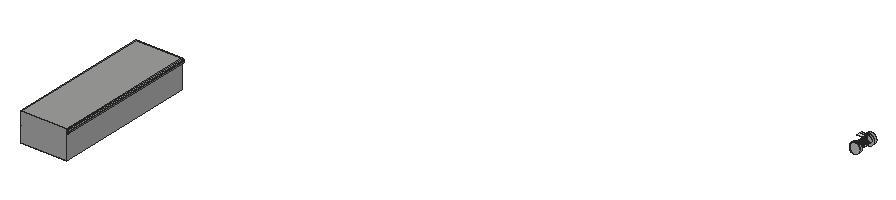
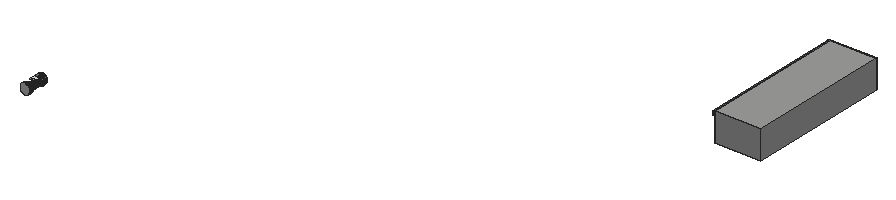
# SketchUp Ruby script. Lengths in inches.
U = 1.inch
M = Sketchup.active_model
def pt(a) = Geom::Point3d.new(a.map { |v| v * U })
def face(e, loops, mat)
  f = e.add_face(loops[0].map { |a| pt(a) })
  loops[1..].each { |l| e.add_face(l.map { |a| pt(a) }).erase! }
  f.material = f.back_material = mat if mat
  f
end
# faces: each face lists its corners as indices into pts; further lists are holes
def faces(e, pts, list, mat = nil) = list.each { |f| face(e, (f[0].is_a?(Array) ? f : [f]).map { |l| l.map { |i| pts[i] } }, mat) }
# xy, xz, yz: faces in a plane at the given z, y or x. An outline is a flat list of corners, or four numbers for a rectangle; further outlines are holes
def ring(l) = l.size == 4 ? [[l[0], l[1]], [l[2], l[1]], [l[2], l[3]], [l[0], l[3]]] : l.each_slice(2).to_a
def flat(e, list, mat, &to3) = list.each { |f| face(e, (f[0].is_a?(Array) ? f : [f]).map { |l| ring(l).map { |u, v| to3.(u, v) } }, mat) }
def xy(e, z, list, mat = nil) = flat(e, list, mat) { |x, y| [x, y, z] }
def xz(e, y, list, mat = nil) = flat(e, list, mat) { |x, z| [x, y, z] }
def yz(e, x, list, mat = nil) = flat(e, list, mat) { |y, z| [x, y, z] }
def lines(e, pts, list) = list.each { |a, b| e.add_line(pt(pts[a]), pt(pts[b])) }
# prism: a flat outline (further loops are holes) pulled along v
def prism(e, loops, v, mat = nil)
  f = face(e, loops, mat); d = Geom::Vector3d.new(v.map { |x| x * U })
  f.pushpull(f.normal.samedirection?(d) ? d.length : -d.length)
end
def box(e, o, s, mat = nil) = prism(e, [[o, [o[0] + s[0], o[1], o[2]], [o[0] + s[0], o[1] + s[1], o[2]], [o[0], o[1] + s[1], o[2]]]], [0, 0, s[2]], mat)
def at(x, y, z, deg = 0) = Geom::Transformation.translation(pt([x, y, z])) * Geom::Transformation.rotation(ORIGIN, Z_AXIS, deg.degrees)
def axes(o, x, y, z) = Geom::Transformation.new([*x, 0, *y, 0, *z, 0, *pt(o).to_a, 1])
def part(name) = M.definitions.add(name)
# library, detail: a bought-in or finely detailed component or shape, given as its bounding box
def library(name, o, s) = part(name).tap { |d| box(d.entities, o, s) }
def detail(e, o, s) = box(e.add_group.entities, o, s)
def put(e, d, t, mat = nil) = e.add_instance(d, t).tap { |i| i.material = mat if mat }
def group(e, t, mat = nil) = e.add_group.tap { |g| g.transformation = t; g.material = mat if mat }.entities
root = M.entities
M.materials.add("[Aluminum]").color = [178, 178, 178]
M.materials.add("crushed-stone-asphalt-staggered-isosceles-2423-mm-architextu").color = [158, 158, 157]
c1 = part("Stair tread")
xy(c1.entities,0,[[0,0,11.5,36]])
xy(c1.entities,7,[[0,0,11.5,36]])
xz(c1.entities,0,[[0,0,11.5,7],[11.5,6,11.63,6.02,11.75,6.07,11.85,6.15,11.93,6.25,11.98,6.37,12,6.5,11.98,6.63,11.93,6.75,11.85,6.85,11.75,6.93,11.63,6.98,11.5,7]])
xz(c1.entities,36,[[0,0,11.5,7],[11.5,6,11.5,7,11.63,6.98,11.75,6.93,11.85,6.85,11.93,6.75,11.98,6.63,12,6.5,11.98,6.37,11.93,6.25,11.85,6.15,11.75,6.07,11.63,6.02]])
yz(c1.entities,0,[[0,0,36,7]])
yz(c1.entities,11.5,[[0,0,36,6],[0,6,10.3125,7],[10.3125,6,36,7]])
p = [[11.5,36,6],[11.63,36,6.02],[11.63,0,6.02],[11.5,0,6],[11.5,10.3125,6],[11.75,36,6.07],
  [11.75,0,6.07],[11.85,36,6.15],[11.85,0,6.15],[11.93,36,6.25],[11.93,0,6.25],[11.98,36,6.37],
  [11.98,0,6.37],[12,36,6.5],[12,0,6.5],[11.98,36,6.63],[11.98,0,6.63],[11.93,36,6.75],
  [11.93,0,6.75],[11.85,36,6.85],[11.85,0,6.85],[11.75,36,6.93],[11.63,36,6.98],[11.63,0,6.98],
  [11.75,0,6.93],[11.5,36,7],[11.5,10.3125,7],[11.5,0,7]]
faces(c1.entities,p,[[0,1,2,3,4],[1,5,6,2],[5,7,8,6],[7,9,10,8],[9,11,12,10],[11,13,14,12],[13,15,16,14],[15,17,18,16],
  [17,19,20,18],[21,22,23,24],[19,21,24,20],[25,26,27,23,22]])
xy(root,65.29,[[211.63,132.28,211.71,133.02]],"[Aluminum]")
xy(root,65.33,[[211.63,127.79,211.71,128.53]],"[Aluminum]")
xy(root,65.58,[[211.65,129.28,211.71,131.53]])
xy(root,65.58,[[211.65,128.53,211.71,129.28],[211.65,131.53,211.71,132.28]],"[Aluminum]")
xy(root,67.55,[[211.65,129.28,211.71,131.53]])
xy(root,67.55,[[211.65,128.53,211.71,129.28],[211.65,131.53,211.71,132.28]],"[Aluminum]")
xy(root,67.8,[[211.63,127.79,211.71,128.53]],"[Aluminum]")
xy(root,67.84,[[211.63,132.28,211.71,133.02]],"[Aluminum]")
xy(root,68.11,[[210.46,130.03,211.84,131.15]])
xy(root,68.11,[[210.46,131.15,211.84,131.53]],"[Aluminum]")
xz(root,127.79,[[211.63,65.33,211.79,65.33,211.95,65.35,212.03,65.37,212.1,65.39,212.17,65.42,212.25,65.46,212.32,65.5,212.38,65.54,212.45,65.58,212.51,65.64,212.57,65.69,212.62,65.75,212.67,65.8125,212.72,65.88,212.76,65.95,212.79,66.02,212.83,66.09,212.85,66.17,212.875,66.25,212.89,66.32,212.91,66.4,212.92,66.48,212.92,66.65,212.91,66.73,212.89,66.81,212.875,66.88,212.85,66.96,212.83,67.04,212.79,67.11,212.76,67.18,212.71,67.25,212.67,67.32,212.62,67.38,212.51,67.49,212.45,67.54,212.38,67.59,212.3125,67.63,212.24,67.67,212.17,67.71,212.1,67.73,212.02,67.76,211.95,67.78,211.79,67.8,211.63,67.8,211.55,67.79,211.48,67.78,211.4,67.76,211.32,67.73,211.18,67.67,211.04,67.59,210.92,67.49,210.86,67.4375,210.81,67.38,210.76,67.32,210.71,67.25,210.63,67.11,210.6,67.04,210.57,66.96,210.53,66.8,210.51,66.64,210.51,66.48,210.53,66.32,210.55,66.24,210.57,66.17,210.6,66.09,210.63,66.02,210.71,65.88,210.76,65.8125,210.81,65.75,210.86,65.69,210.92,65.63,210.98,65.58,211.04,65.54,211.11,65.49,211.18,65.46,211.25,65.42,211.33,65.39,211.4,65.37,211.48,65.35,211.56,65.34]],"[Aluminum]")
xz(root,128.53,[[[211.63,65.33,211.56,65.34,211.48,65.35,211.4,65.37,211.33,65.39,211.25,65.42,211.18,65.46,211.11,65.49,211.04,65.54,210.98,65.58,210.92,65.63,210.86,65.69,210.81,65.75,210.76,65.8125,210.71,65.88,210.63,66.02,210.6,66.09,210.57,66.17,210.55,66.24,210.53,66.32,210.51,66.48,210.51,66.64,210.53,66.8,210.57,66.96,210.6,67.04,210.63,67.11,210.71,67.25,210.76,67.32,210.81,67.38,210.86,67.4375,210.92,67.49,211.04,67.59,211.18,67.67,211.32,67.73,211.4,67.76,211.48,67.78,211.55,67.79,211.63,67.8,211.79,67.8,211.95,67.78,212.02,67.76,212.1,67.73,212.17,67.71,212.24,67.67,212.3125,67.63,212.38,67.59,212.45,67.54,212.51,67.49,212.62,67.38,212.67,67.32,212.71,67.25,212.76,67.18,212.79,67.11,212.83,67.04,212.85,66.96,212.875,66.88,212.89,66.81,212.91,66.73,212.92,66.65,212.92,66.48,212.91,66.4,212.89,66.32,212.875,66.25,212.85,66.17,212.83,66.09,212.79,66.02,212.76,65.95,212.72,65.88,212.67,65.8125,212.62,65.75,212.57,65.69,212.51,65.64,212.45,65.58,212.38,65.54,212.32,65.5,212.25,65.46,212.17,65.42,212.1,65.39,212.03,65.37,211.95,65.35,211.79,65.33],[211.65,65.58,211.78,65.58,211.96,65.61,212.02,65.63,212.08,65.66,212.14,65.68,212.19,65.71,212.25,65.75,212.3,65.78,212.35,65.82,212.39,65.87,212.44,65.92,212.48,65.97,212.51,66.02,212.55,66.07,212.57,66.13,212.6,66.1875,212.625,66.25,212.64,66.31,212.66,66.37,212.67,66.4375,212.67,66.69,212.66,66.76,212.64,66.82,212.625,66.88,212.6,66.94,212.57,67,212.55,67.06,212.51,67.11,212.48,67.16,212.44,67.21,212.35,67.3,212.25,67.38,212.19,67.42,212.14,67.45,212.08,67.47,212.02,67.5,211.96,67.51,211.9,67.53,211.78,67.55,211.65,67.55,211.53,67.53,211.46,67.51,211.4,67.5,211.34,67.47,211.29,67.45,211.23,67.42,211.03,67.26,210.91,67.11,210.88,67.06,210.82,66.94,210.78,66.82,210.77,66.76,210.76,66.69,210.75,66.63,210.75,66.5,210.76,66.4375,210.77,66.37,210.78,66.31,210.8,66.25,210.82,66.1875,210.85,66.13,210.88,66.07,210.91,66.02,211.03,65.87,211.08,65.82,211.13,65.78,211.18,65.75,211.23,65.71,211.29,65.68,211.34,65.66,211.4,65.63,211.46,65.61,211.53,65.6]]],"[Aluminum]")
xz(root,132.28,[[[211.63,65.29,211.79,65.29,211.96,65.31,212.04,65.33,212.11,65.35,212.19,65.38,212.26,65.42,212.34,65.46,212.41,65.5,212.47,65.55,212.54,65.6,212.6,65.66,212.65,65.72,212.7,65.79,212.75,65.85,212.79,65.93,212.83,66,212.87,66.08,212.89,66.15,212.92,66.23,212.9375,66.31,212.95,66.4,212.96,66.48,212.96,66.65,212.95,66.73,212.9375,66.8125,212.92,66.9,212.89,66.98,212.87,67.05,212.83,67.13,212.75,67.27,212.65,67.41,212.59,67.47,212.54,67.53,212.47,67.58,212.41,67.63,212.34,67.67,212.26,67.71,212.19,67.75,212.11,67.78,212.04,67.8,211.96,67.82,211.79,67.84,211.63,67.84,211.47,67.82,211.39,67.8,211.3125,67.78,211.23,67.75,211.02,67.63,210.95,67.58,210.89,67.53,210.77,67.41,210.67,67.27,210.59,67.13,210.56,67.05,210.53,66.98,210.51,66.89,210.49,66.8125,210.48,66.73,210.47,66.65,210.46,66.5625,210.47,66.48,210.48,66.4,210.49,66.3125,210.51,66.23,210.53,66.15,210.56,66.07,210.59,66,210.63,65.92,210.68,65.85,210.72,65.79,210.77,65.72,210.89,65.6,210.95,65.55,211.02,65.5,211.16,65.42,211.24,65.38,211.3125,65.35,211.39,65.33,211.47,65.31],[211.65,65.58,211.53,65.6,211.46,65.61,211.4,65.63,211.34,65.66,211.29,65.68,211.23,65.71,211.18,65.75,211.13,65.78,211.08,65.82,211.03,65.87,210.91,66.02,210.88,66.07,210.85,66.13,210.82,66.1875,210.8,66.25,210.78,66.31,210.77,66.37,210.76,66.4375,210.75,66.5,210.75,66.63,210.76,66.69,210.77,66.76,210.78,66.82,210.82,66.94,210.88,67.06,210.91,67.11,211.03,67.26,211.23,67.42,211.29,67.45,211.34,67.47,211.4,67.5,211.46,67.51,211.53,67.53,211.65,67.55,211.78,67.55,211.9,67.53,211.96,67.51,212.02,67.5,212.08,67.47,212.14,67.45,212.19,67.42,212.25,67.38,212.35,67.3,212.44,67.21,212.48,67.16,212.51,67.11,212.55,67.06,212.57,67,212.6,66.94,212.625,66.88,212.64,66.82,212.66,66.76,212.67,66.69,212.67,66.4375,212.66,66.37,212.64,66.31,212.625,66.25,212.6,66.1875,212.57,66.13,212.55,66.07,212.51,66.02,212.48,65.97,212.44,65.92,212.39,65.87,212.35,65.82,212.3,65.78,212.25,65.75,212.19,65.71,212.14,65.68,212.08,65.66,212.02,65.63,211.96,65.61,211.78,65.58]]],"[Aluminum]")
xz(root,133.02,[[211.63,65.29,211.47,65.31,211.39,65.33,211.3125,65.35,211.24,65.38,211.16,65.42,211.02,65.5,210.95,65.55,210.89,65.6,210.77,65.72,210.72,65.79,210.68,65.85,210.63,65.92,210.59,66,210.56,66.07,210.53,66.15,210.51,66.23,210.49,66.3125,210.48,66.4,210.47,66.48,210.46,66.5625,210.47,66.65,210.48,66.73,210.49,66.8125,210.51,66.89,210.53,66.98,210.56,67.05,210.59,67.13,210.67,67.27,210.77,67.41,210.89,67.53,210.95,67.58,211.02,67.63,211.23,67.75,211.3125,67.78,211.39,67.8,211.47,67.82,211.63,67.84,211.79,67.84,211.96,67.82,212.04,67.8,212.11,67.78,212.19,67.75,212.26,67.71,212.34,67.67,212.41,67.63,212.47,67.58,212.54,67.53,212.59,67.47,212.65,67.41,212.75,67.27,212.83,67.13,212.87,67.05,212.89,66.98,212.92,66.9,212.9375,66.8125,212.95,66.73,212.96,66.65,212.96,66.48,212.95,66.4,212.9375,66.31,212.92,66.23,212.89,66.15,212.87,66.08,212.83,66,212.79,65.93,212.75,65.85,212.7,65.79,212.65,65.72,212.6,65.66,212.54,65.6,212.47,65.55,212.41,65.5,212.34,65.46,212.26,65.42,212.19,65.38,212.11,65.35,212.04,65.33,211.96,65.31,211.79,65.29]],"[Aluminum]")
yz(root,210.51,[[127.79,66.48,128.53,66.5625],[127.79,66.5625,128.53,66.64]],"[Aluminum]")
yz(root,210.75,[[129.28,66.5,131.53,66.5625],[129.28,66.5625,131.53,66.63]])
yz(root,210.75,[[128.53,66.5,129.28,66.5625],[131.53,66.5,132.28,66.5625],[128.53,66.5625,129.28,66.63],[131.53,66.5625,132.28,66.63]],"[Aluminum]")
p = [[211.48,128.53,65.35],[211.56,128.53,65.34],[211.56,127.79,65.34],[211.48,127.79,65.35],[211.63,128.53,65.33],[211.63,127.79,65.33],
  [211.39,132.28,65.33],[211.3125,132.28,65.35],[211.3125,133.02,65.35],[211.39,133.02,65.33],[211.47,132.28,65.31],[211.47,133.02,65.31],
  [211.55,132.28,65.3],[211.55,133.02,65.3],[211.63,132.28,65.29],[211.63,133.02,65.29],[211.18,128.53,65.46],[211.25,128.53,65.42],
  [211.25,127.79,65.42],[211.18,127.79,65.46],[211.33,128.53,65.39],[211.33,127.79,65.39],[211.4,128.53,65.37],[211.4,127.79,65.37],
  [211.16,132.28,65.42],[211.09,132.28,65.46],[211.09,133.02,65.46],[211.16,133.02,65.42],[211.24,132.28,65.38],[211.24,133.02,65.38],
  [210.98,128.53,65.58],[211.04,128.53,65.54],[211.04,127.79,65.54],[210.98,127.79,65.58],[211.11,128.53,65.49],[211.11,127.79,65.49],
  [210.95,132.28,65.55],[210.89,132.28,65.6],[210.89,133.02,65.6],[210.95,133.02,65.55],[211.02,132.28,65.5],[211.02,133.02,65.5],
  [210.86,128.53,65.69],[210.92,128.53,65.63],[210.92,127.79,65.63],[210.86,127.79,65.69],[211.4,129.28,65.63],[211.34,129.28,65.66],
  [211.34,128.53,65.66],[211.4,128.53,65.63],[211.46,129.28,65.61],[211.46,128.53,65.61],[211.53,129.28,65.6],[211.53,128.53,65.6],
  [211.59,129.28,65.59],[211.59,128.53,65.59],[211.65,129.28,65.58],[211.65,128.53,65.58],[211.34,131.53,65.66],[211.4,131.53,65.63],
  [211.46,131.53,65.61],[211.53,131.53,65.6],[211.59,131.53,65.59],[211.65,131.53,65.58],[211.34,132.28,65.66],[211.4,132.28,65.63],
  [211.46,132.28,65.61],[211.53,132.28,65.6],[211.59,132.28,65.59],[211.65,132.28,65.58],[210.83,132.28,65.66],[210.83,133.02,65.66],
  [210.76,128.53,65.8125],[210.81,128.53,65.75],[210.81,127.79,65.75],[210.76,127.79,65.8125],[211.18,129.28,65.75],[211.13,129.28,65.78],
  [211.13,128.53,65.78],[211.18,128.53,65.75],[211.23,129.28,65.71],[211.23,128.53,65.71],[211.29,129.28,65.68],[211.29,128.53,65.68],
  [211.13,131.53,65.78],[211.18,131.53,65.75],[211.23,131.53,65.71],[211.29,131.53,65.68],[211.13,132.28,65.78],[211.18,132.28,65.75],
  [211.23,132.28,65.71],[211.29,132.28,65.68],[210.77,132.28,65.72],[210.72,132.28,65.79],[210.72,133.02,65.79],[210.77,133.02,65.72],
  [210.71,128.53,65.88],[210.71,127.79,65.88],[211.08,129.28,65.82],[211.03,129.28,65.87],[211.03,128.53,65.87],[211.08,128.53,65.82],
  [211.03,131.53,65.87],[211.08,131.53,65.82],[211.03,132.28,65.87],[211.08,132.28,65.82],[210.68,132.28,65.85],[210.68,133.02,65.85],
  [210.63,128.53,66.02],[210.67,128.53,65.95],[210.67,127.79,65.95],[210.63,127.79,66.02],[210.99,129.28,65.92],[210.95,129.28,65.97],
  [210.95,128.53,65.97],[210.99,128.53,65.92],[210.95,131.53,65.97],[210.99,131.53,65.92],[210.95,132.28,65.97],[210.99,132.28,65.92],
  [210.63,132.28,65.92],[210.59,132.28,66],[210.59,133.02,66],[210.63,133.02,65.92],[210.6,128.53,66.09],[210.6,127.79,66.09],
  [210.91,129.28,66.02],[210.88,129.28,66.07],[210.88,128.53,66.07],[210.91,128.53,66.02],[210.88,131.53,66.07],[210.91,131.53,66.02],
  [210.88,132.28,66.07],[210.91,132.28,66.02],[210.56,132.28,66.07],[210.56,133.02,66.07],[210.57,128.53,66.17],[210.57,127.79,66.17],
  [210.85,129.28,66.13],[210.82,129.28,66.1875],[210.82,128.53,66.1875],[210.85,128.53,66.13],[210.82,131.53,66.1875],[210.85,131.53,66.13],
  [210.82,132.28,66.1875],[210.85,132.28,66.13],[210.53,132.28,66.15],[210.53,133.02,66.15],[210.53,128.53,66.32],[210.55,128.53,66.24],
  [210.55,127.79,66.24],[210.53,127.79,66.32],[210.8,129.28,66.25],[210.78,129.28,66.31],[210.78,128.53,66.31],[210.8,128.53,66.25],
  [210.78,131.53,66.31],[210.8,131.53,66.25],[210.78,132.28,66.31],[210.8,132.28,66.25],[210.51,132.28,66.23],[210.49,132.28,66.3125],
  [210.49,133.02,66.3125],[210.51,133.02,66.23],[210.52,128.53,66.4],[210.52,127.79,66.4],[210.77,129.28,66.37],[210.77,128.53,66.37],
  [210.77,131.53,66.37],[210.77,132.28,66.37],[210.48,132.28,66.4],[210.48,133.02,66.4],[210.51,128.53,66.48],[210.51,127.79,66.48],
  [210.76,129.28,66.4375],[210.75,129.28,66.5],[210.75,128.53,66.5],[210.76,128.53,66.4375],[210.75,131.53,66.5],[210.76,131.53,66.4375],
  [210.75,132.28,66.5],[210.76,132.28,66.4375],[210.47,132.28,66.48],[210.47,133.02,66.48],[210.46,132.28,66.5625],[210.46,133.02,66.5625],
  [210.52,128.53,66.72],[210.51,128.53,66.64],[210.51,127.79,66.64],[210.52,127.79,66.72],[210.75,129.28,66.63],[210.76,129.28,66.69],
  [210.76,128.53,66.69],[210.75,128.53,66.63],[210.76,131.53,66.69],[210.75,131.53,66.63],[210.76,132.28,66.69],[210.75,132.28,66.63],
  [210.47,132.28,66.65],[210.47,133.02,66.65],[210.48,132.28,66.73],[210.48,133.02,66.73],[210.53,128.53,66.8],[210.53,127.79,66.8],
  [210.77,129.28,66.76],[210.77,128.53,66.76],[210.77,131.53,66.76],[210.77,132.28,66.76],[210.49,132.28,66.8125],[210.49,133.02,66.8125],
  [210.55,128.53,66.88],[210.55,127.79,66.88],[210.78,129.28,66.82],[210.78,128.53,66.82],[210.8,129.28,66.88],[210.8,128.53,66.88],
  [210.78,131.53,66.82],[210.8,131.53,66.88],[210.78,132.28,66.82],[210.8,132.28,66.88],[210.51,132.28,66.89],[210.51,133.02,66.89],
  [210.57,128.53,66.96],[210.57,127.79,66.96],[210.82,129.28,66.94],[210.82,128.53,66.94],[210.85,129.28,67],[210.85,128.53,67],
  [210.82,131.53,66.94],[210.85,131.53,67],[210.82,132.28,66.94],[210.85,132.28,67],[210.53,132.28,66.98],[210.53,133.02,66.98],
  [210.6,128.53,67.04],[210.6,127.79,67.04],[210.63,128.53,67.11],[210.63,127.79,67.11],[210.88,129.28,67.06],[210.88,128.53,67.06],
  [210.88,131.53,67.06],[210.88,132.28,67.06],[210.56,132.28,67.05],[210.56,133.02,67.05],[210.67,128.53,67.18],[210.67,127.79,67.18],
  [210.91,129.28,67.11],[210.91,128.53,67.11],[210.95,129.28,67.16],[210.95,128.53,67.16],[210.91,131.53,67.11],[210.95,131.53,67.16],
  [210.91,132.28,67.11],[210.95,132.28,67.16],[210.59,132.28,67.13],[210.59,133.02,67.13],[210.63,132.28,67.2],[210.63,133.02,67.2],
  [210.71,128.53,67.25],[210.71,127.79,67.25],[210.76,128.53,67.32],[210.76,127.79,67.32],[210.99,129.28,67.21],[210.99,128.53,67.21],
  [211.03,129.28,67.26],[211.03,128.53,67.26],[210.99,131.53,67.21],[211.03,131.53,67.26],[210.99,132.28,67.21],[211.03,132.28,67.26],
  [210.67,132.28,67.27],[210.67,133.02,67.27],[210.81,128.53,67.38],[210.81,127.79,67.38],[211.08,129.28,67.3],[211.08,128.53,67.3],
  [211.13,129.28,67.34],[211.13,128.53,67.34],[211.18,129.28,67.38],[211.18,128.53,67.38],[211.08,131.53,67.3],[211.13,131.53,67.34],
  [211.18,131.53,67.38],[211.08,132.28,67.3],[211.13,132.28,67.34],[211.18,132.28,67.38],[210.72,132.28,67.34],[210.72,133.02,67.34],
  [210.77,132.28,67.41],[210.77,133.02,67.41],[210.86,128.53,67.4375],[210.86,127.79,67.4375],[210.92,128.53,67.49],[210.92,127.79,67.49],
  [211.23,129.28,67.42],[211.23,128.53,67.42],[211.29,129.28,67.45],[211.29,128.53,67.45],[211.34,129.28,67.47],[211.34,128.53,67.47],
  [211.23,131.53,67.42],[211.29,131.53,67.45],[211.34,131.53,67.47],[211.23,132.28,67.42],[211.29,132.28,67.45],[211.34,132.28,67.47],
  [210.83,132.28,67.47],[210.83,133.02,67.47],[210.98,128.53,67.54],[210.98,127.79,67.54],[211.04,128.53,67.59],[211.04,127.79,67.59],
  [211.4,129.28,67.5],[211.4,128.53,67.5],[211.46,129.28,67.51],[211.46,128.53,67.51],[211.53,129.28,67.53],[211.53,128.53,67.53],
  [211.59,129.28,67.54],[211.59,128.53,67.54],[211.65,129.28,67.55],[211.65,128.53,67.55],[211.4,131.53,67.5],[211.46,131.53,67.51],
  [211.53,131.53,67.53],[211.59,131.53,67.54],[211.65,131.53,67.55],[211.4,132.28,67.5],[211.46,132.28,67.51],[211.53,132.28,67.53],
  [211.59,132.28,67.54],[211.65,132.28,67.55],[210.89,132.28,67.53],[210.89,133.02,67.53],[210.95,132.28,67.58],[210.95,133.02,67.58],
  [211.11,128.53,67.63],[211.11,127.79,67.63],[211.18,128.53,67.67],[211.18,127.79,67.67],[211.02,132.28,67.63],[211.02,133.02,67.63],
  [211.09,132.28,67.67],[211.09,133.02,67.67],[211.25,128.53,67.7],[211.25,127.79,67.7],[211.32,128.53,67.73],[211.32,127.79,67.73],
  [211.4,128.53,67.76],[211.4,127.79,67.76],[211.16,132.28,67.71],[211.16,133.02,67.71],[211.23,132.28,67.75],[211.23,133.02,67.75],
  [211.3125,132.28,67.78],[211.3125,133.02,67.78],[211.48,128.53,67.78],[211.48,127.79,67.78],[211.55,128.53,67.79],[211.55,127.79,67.79],
  [211.63,128.53,67.8],[211.63,127.79,67.8],[211.39,132.28,67.8],[211.39,133.02,67.8],[211.47,132.28,67.82],[211.47,133.02,67.82],
  [211.55,132.28,67.83],[211.55,133.02,67.83],[211.63,132.28,67.84],[211.63,133.02,67.84]]
faces(root,p,[[0,1,2,3],[1,4,5,2],[6,7,8,9],[10,6,9,11],[12,10,11,13],[14,12,13,15],[16,17,18,19],[17,20,21,18],
  [20,22,23,21],[22,0,3,23],[24,25,26,27],[28,24,27,29],[7,28,29,8],[30,31,32,33],[31,34,35,32],[34,16,19,35],
  [36,37,38,39],[40,36,39,41],[25,40,41,26],[42,43,44,45],[43,30,33,44],[46,47,48,49],[50,46,49,51],[52,50,51,53],
  [54,52,53,55],[56,54,55,57],[59,58,64,65],[60,59,65,66],[61,60,66,67],[62,61,67,68],[63,62,68,69],[37,70,71,38],
  [72,73,74,75],[73,42,45,74],[76,77,78,79],[80,76,79,81],[82,80,81,83],[47,82,83,48],[85,84,88,89],[86,85,89,90],
  [87,86,90,91],[58,87,91,64],[92,93,94,95],[70,92,95,71],[96,72,75,97],[98,99,100,101],[77,98,101,78],[103,102,104,105],
  [84,103,105,88],[93,106,107,94],[108,109,110,111],[109,96,97,110],[112,113,114,115],[99,112,115,100],[117,116,118,119],[102,117,119,104],
  [120,121,122,123],[106,120,123,107],[124,108,111,125],[126,127,128,129],[113,126,129,114],[131,130,132,133],[116,131,133,118],[121,134,135,122],
  [136,124,125,137],[138,139,140,141],[127,138,141,128],[143,142,144,145],[130,143,145,132],[134,146,147,135],[148,149,150,151],[149,136,137,150],
  [152,153,154,155],[139,152,155,140],[157,156,158,159],[142,157,159,144],[160,161,162,163],[146,160,163,147],[164,148,151,165],[153,166,167,154],
  [156,168,169,158],[161,170,171,162],[172,164,165,173],[174,175,176,177],[166,174,177,167],[179,178,180,181],[168,179,181,169],[170,182,183,171],
  [182,184,185,183],[186,187,188,189],[190,191,192,193],[195,194,196,197],[184,198,199,185],[198,200,201,199],[202,186,189,203],[191,204,205,192],
  [194,206,207,196],[200,208,209,201],[210,202,203,211],[204,212,213,205],[212,214,215,213],[206,216,218,207],[216,217,219,218],[208,220,221,209],
  [222,210,211,223],[214,224,225,215],[224,226,227,225],[217,228,230,219],[228,229,231,230],[220,232,233,221],[234,222,223,235],[236,234,235,237],
  [226,238,239,227],[229,240,241,231],[232,242,243,233],[244,236,237,245],[238,246,247,239],[246,248,249,247],[240,250,252,241],[250,251,253,252],
  [242,254,255,243],[254,256,257,255],[258,244,245,259],[260,258,259,261],[248,262,263,249],[262,264,265,263],[251,266,268,253],[266,267,269,268],
  [256,270,271,257],[272,260,261,273],[264,274,275,265],[274,276,277,275],[276,278,279,277],[267,280,283,269],[280,281,284,283],[281,282,285,284],
  [270,286,287,271],[286,288,289,287],[290,272,273,291],[292,290,291,293],[278,294,295,279],[294,296,297,295],[296,298,299,297],[282,300,303,285],
  [300,301,304,303],[301,302,305,304],[288,306,307,289],[308,292,293,309],[310,308,309,311],[298,312,313,299],[312,314,315,313],[314,316,317,315],
  [316,318,319,317],[318,320,321,319],[302,322,327,305],[322,323,328,327],[323,324,329,328],[324,325,330,329],[325,326,331,330],[306,332,333,307],
  [332,334,335,333],[336,310,311,337],[338,336,337,339],[334,340,341,335],[340,342,343,341],[344,338,339,345],[346,344,345,347],[348,346,347,349],
  [342,350,351,343],[350,352,353,351],[352,354,355,353],[356,348,349,357],[358,356,357,359],[360,358,359,361],[354,362,363,355],[362,364,365,363],
  [364,366,367,365],[366,368,369,367]],"[Aluminum]")
faces(root,p,[[58,59,46,47],[59,60,50,46],[60,61,52,50],[61,62,54,52],[62,63,56,54],[84,85,76,77],[85,86,80,76],[86,87,82,80],
  [87,58,47,82],[102,103,98,99],[103,84,77,98],[116,117,112,113],[117,102,99,112],[130,131,126,127],[131,116,113,126],[142,143,138,139],
  [143,130,127,138],[156,157,152,153],[157,142,139,152],[168,156,153,166],[178,179,174,175],[179,168,166,174],[194,195,190,191],[206,194,191,204],
  [216,206,204,212],[217,216,212,214],[228,217,214,224],[229,228,224,226],[240,229,226,238],[250,240,238,246],[251,250,246,248],[266,251,248,262],
  [267,266,262,264],[280,267,264,274],[281,280,274,276],[282,281,276,278],[300,282,278,294],[301,300,294,296],[302,301,296,298],[322,302,298,312],
  [323,322,312,314],[324,323,314,316],[325,324,316,318],[326,325,318,320]])
put(root,c1,at(83.05,29.1875,66),"crushed-stone-asphalt-staggered-isosceles-2423-mm-architextu")
